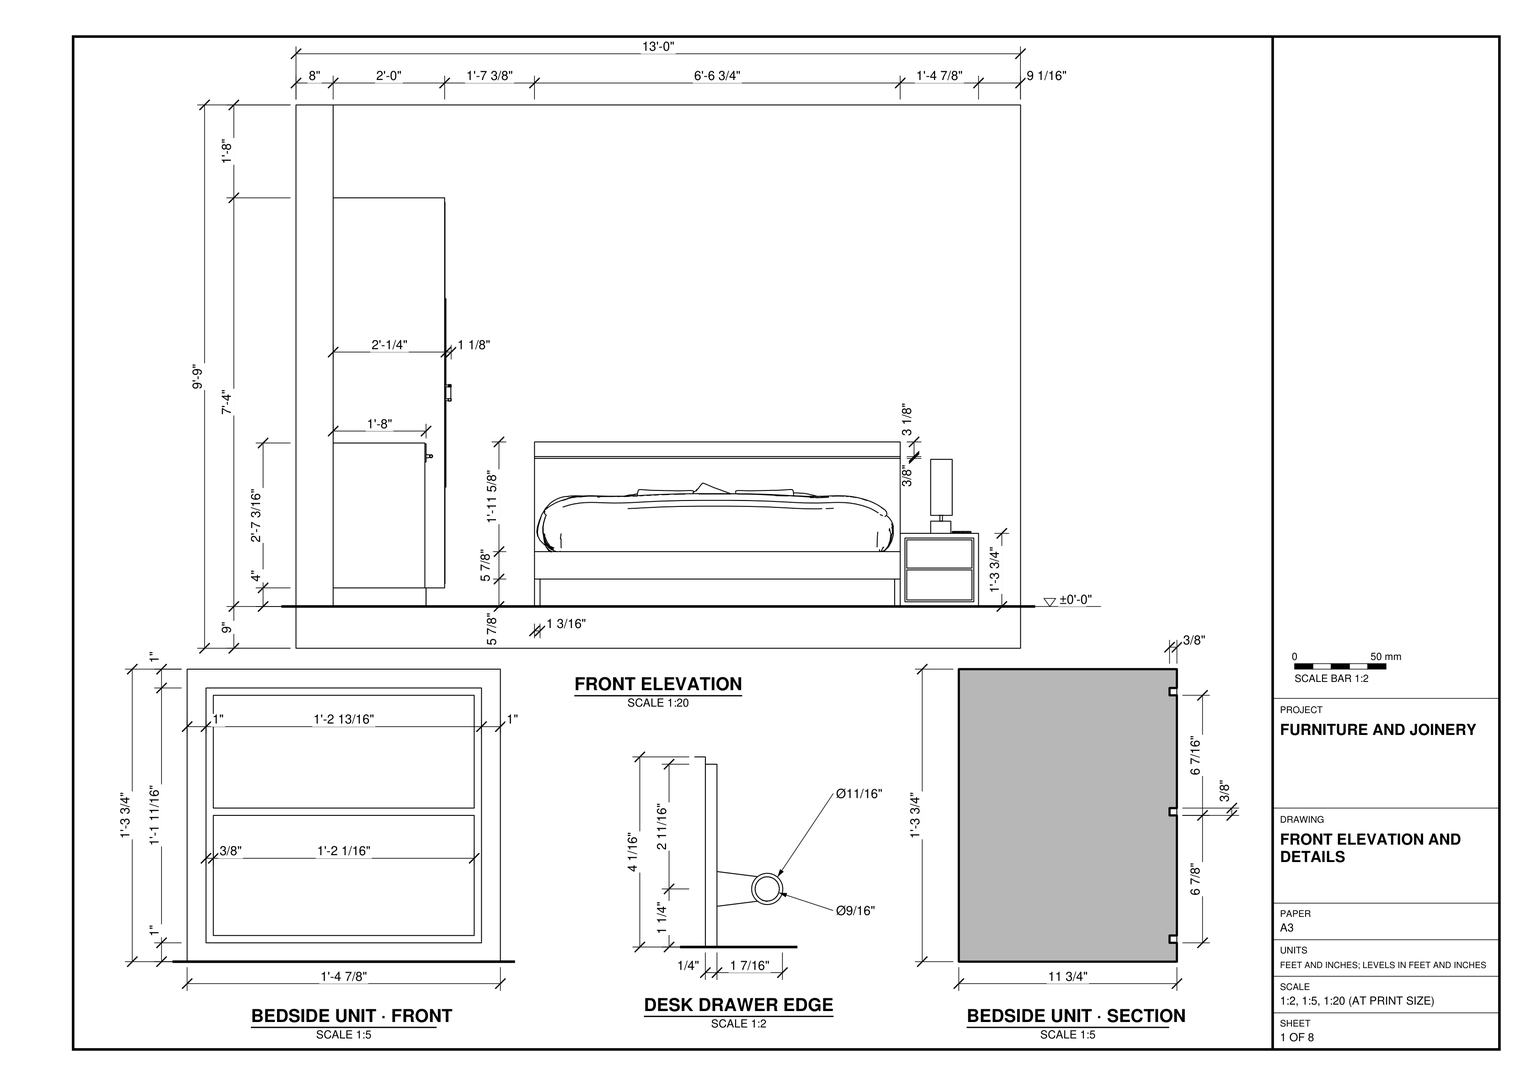
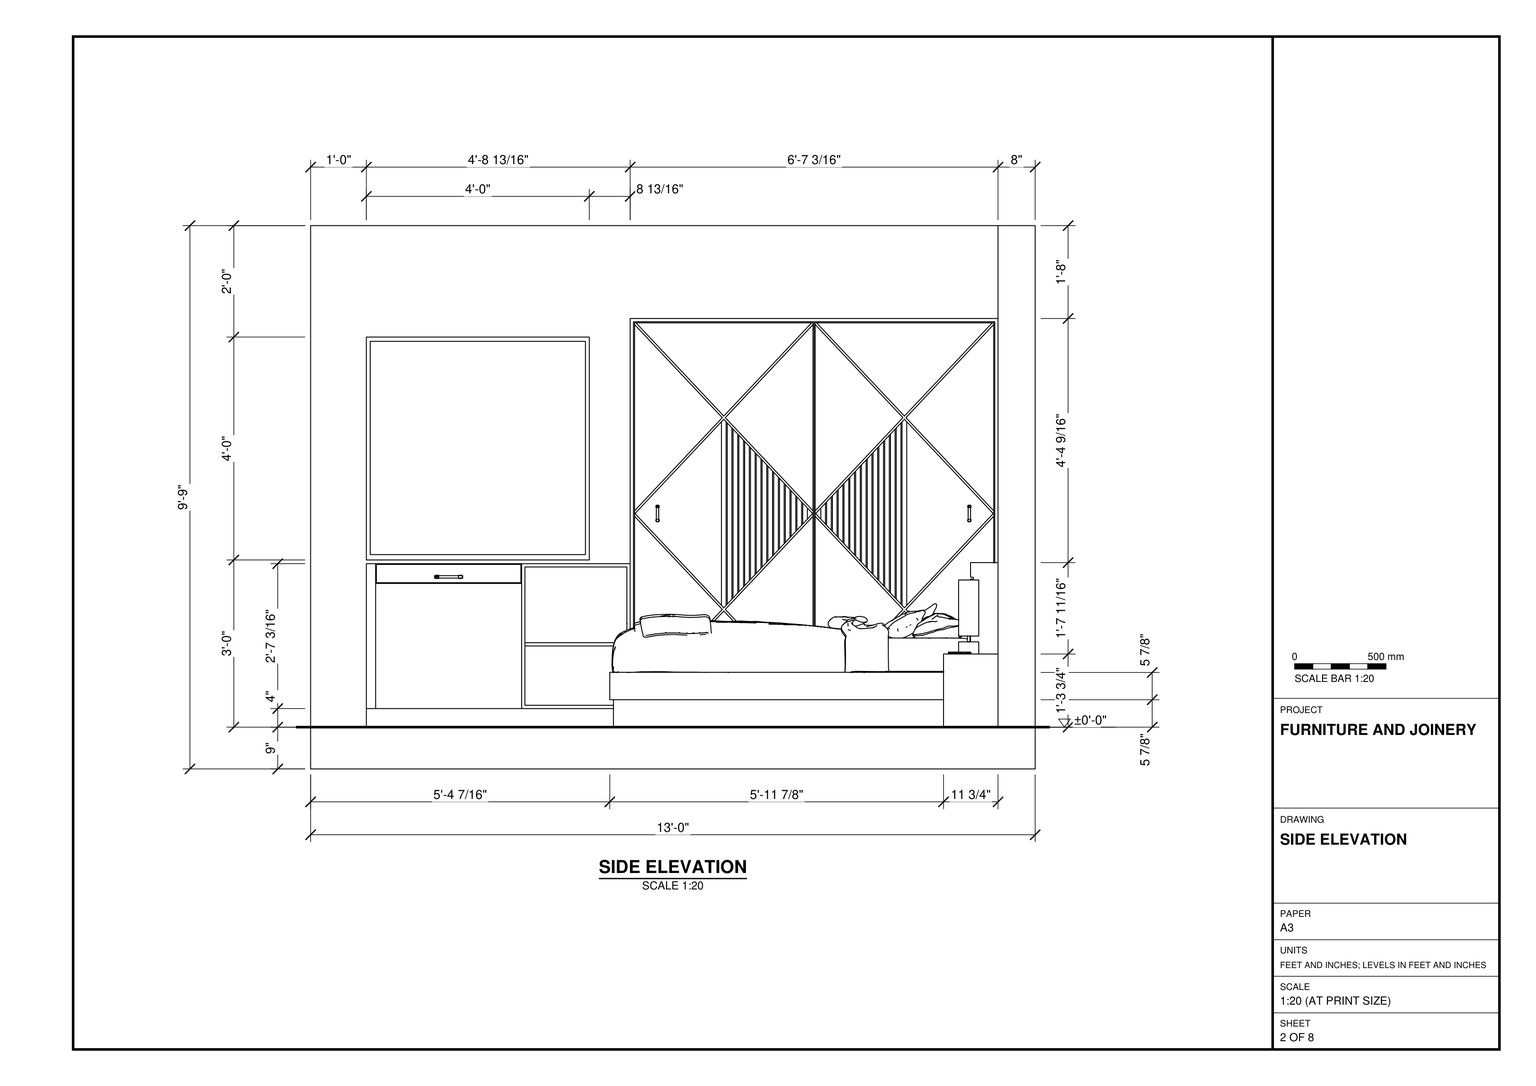
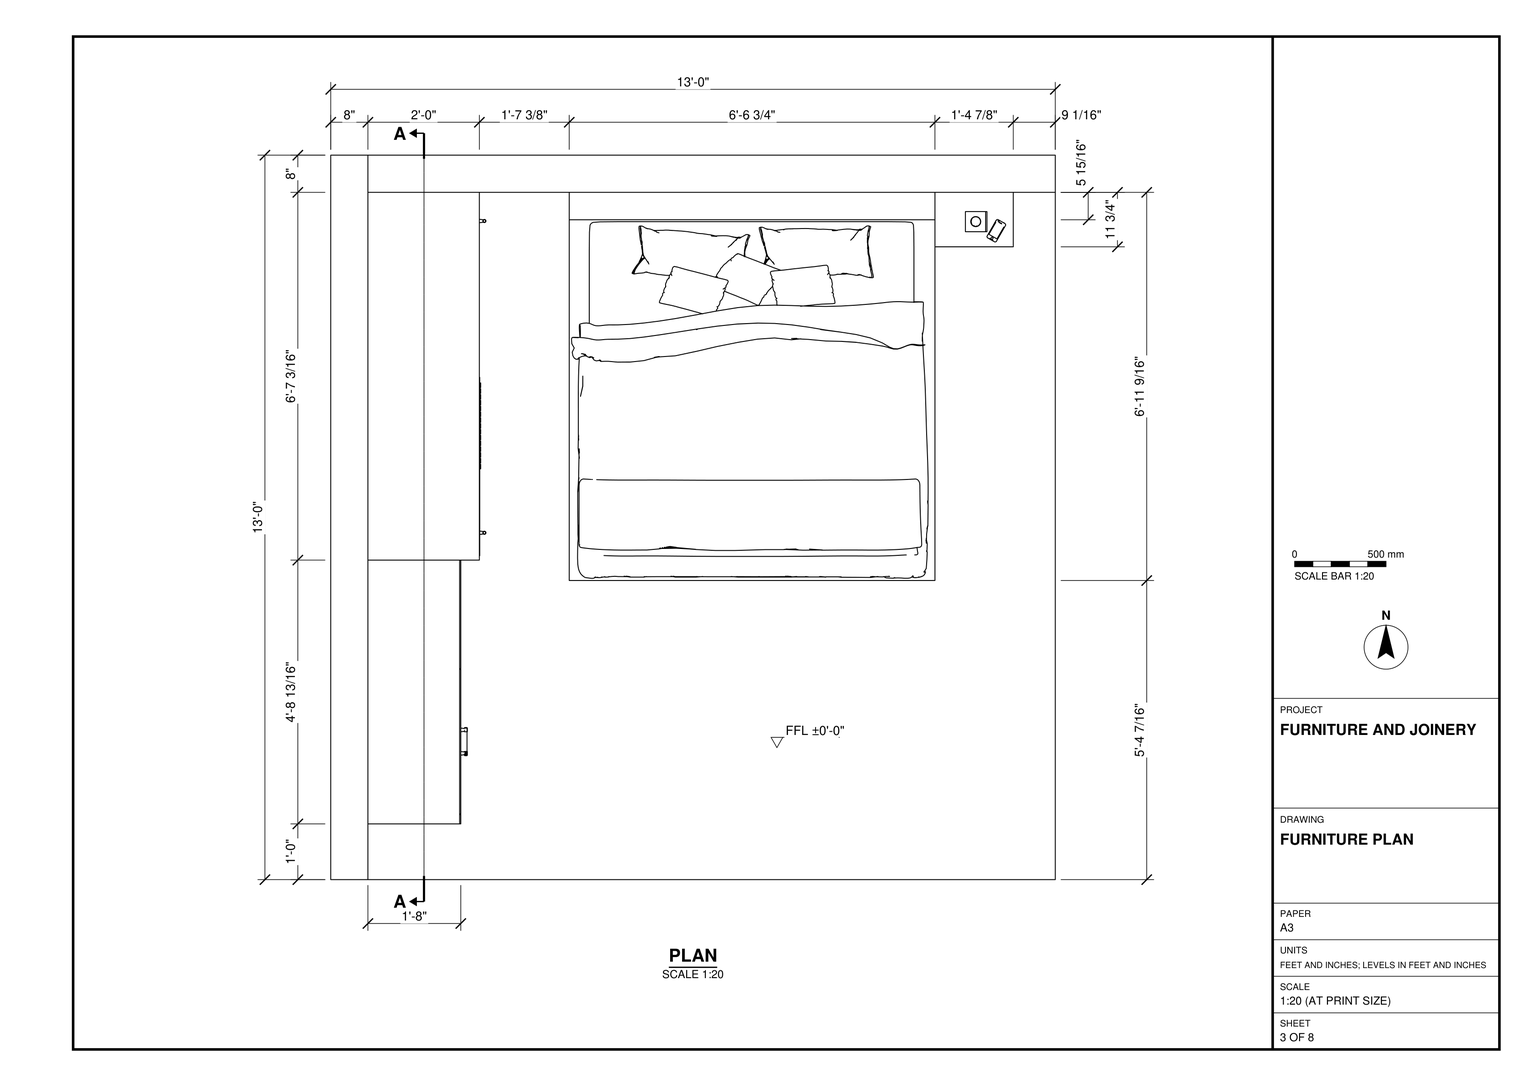
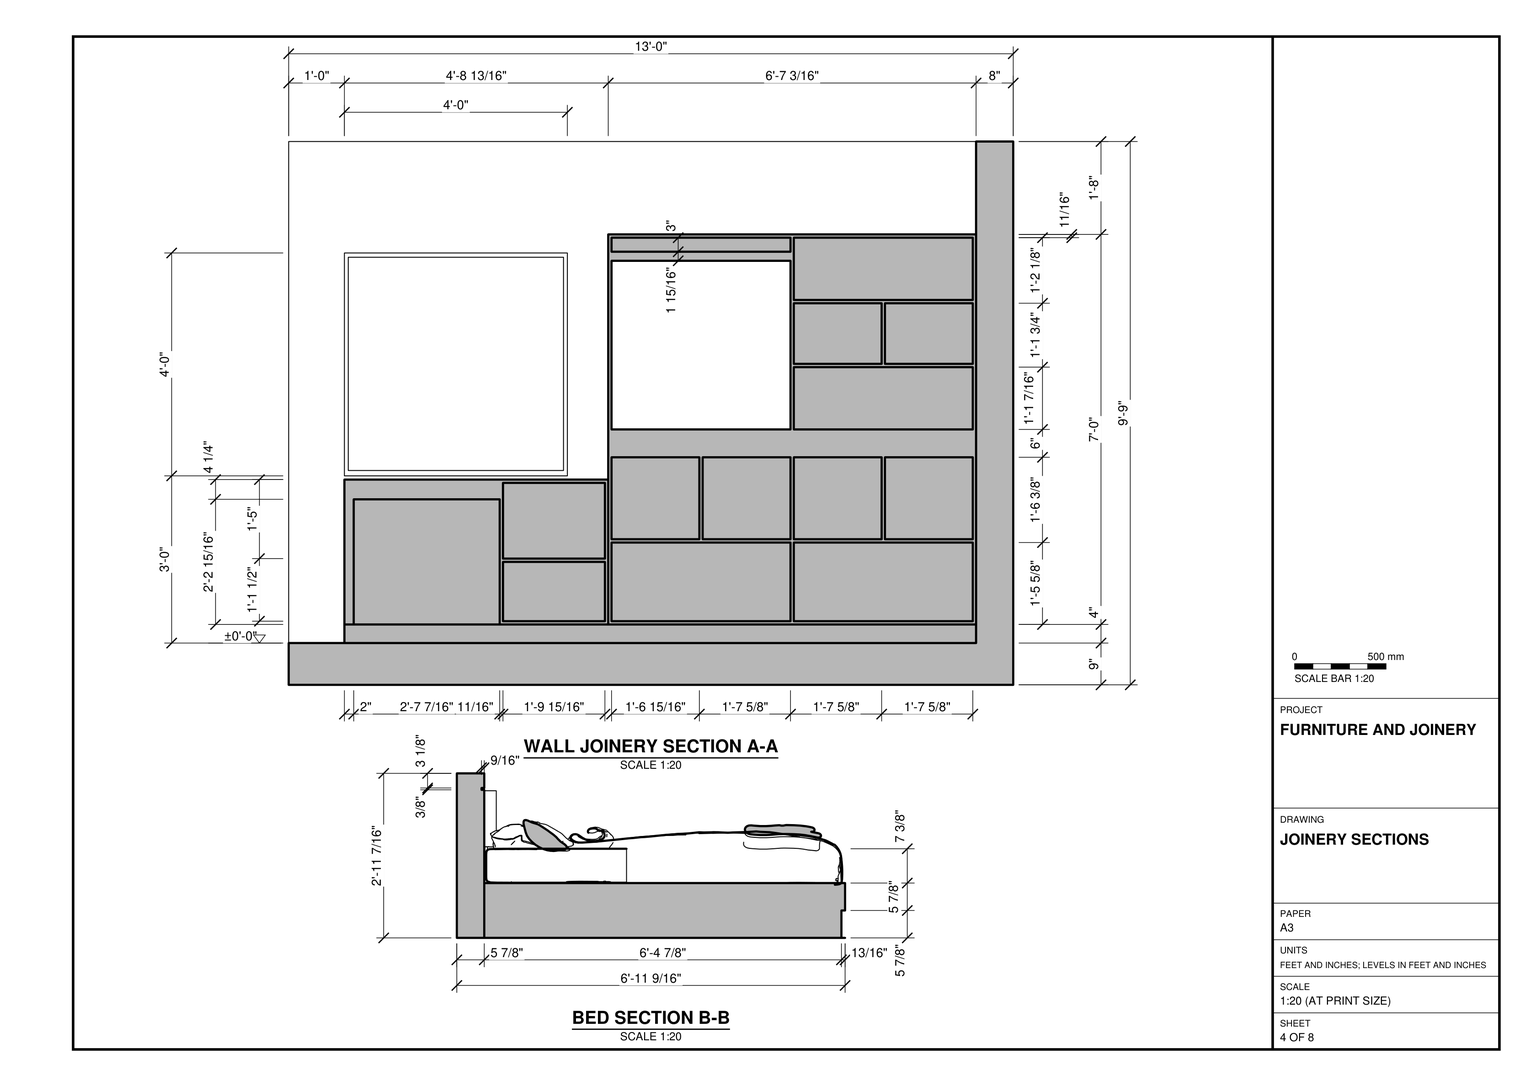
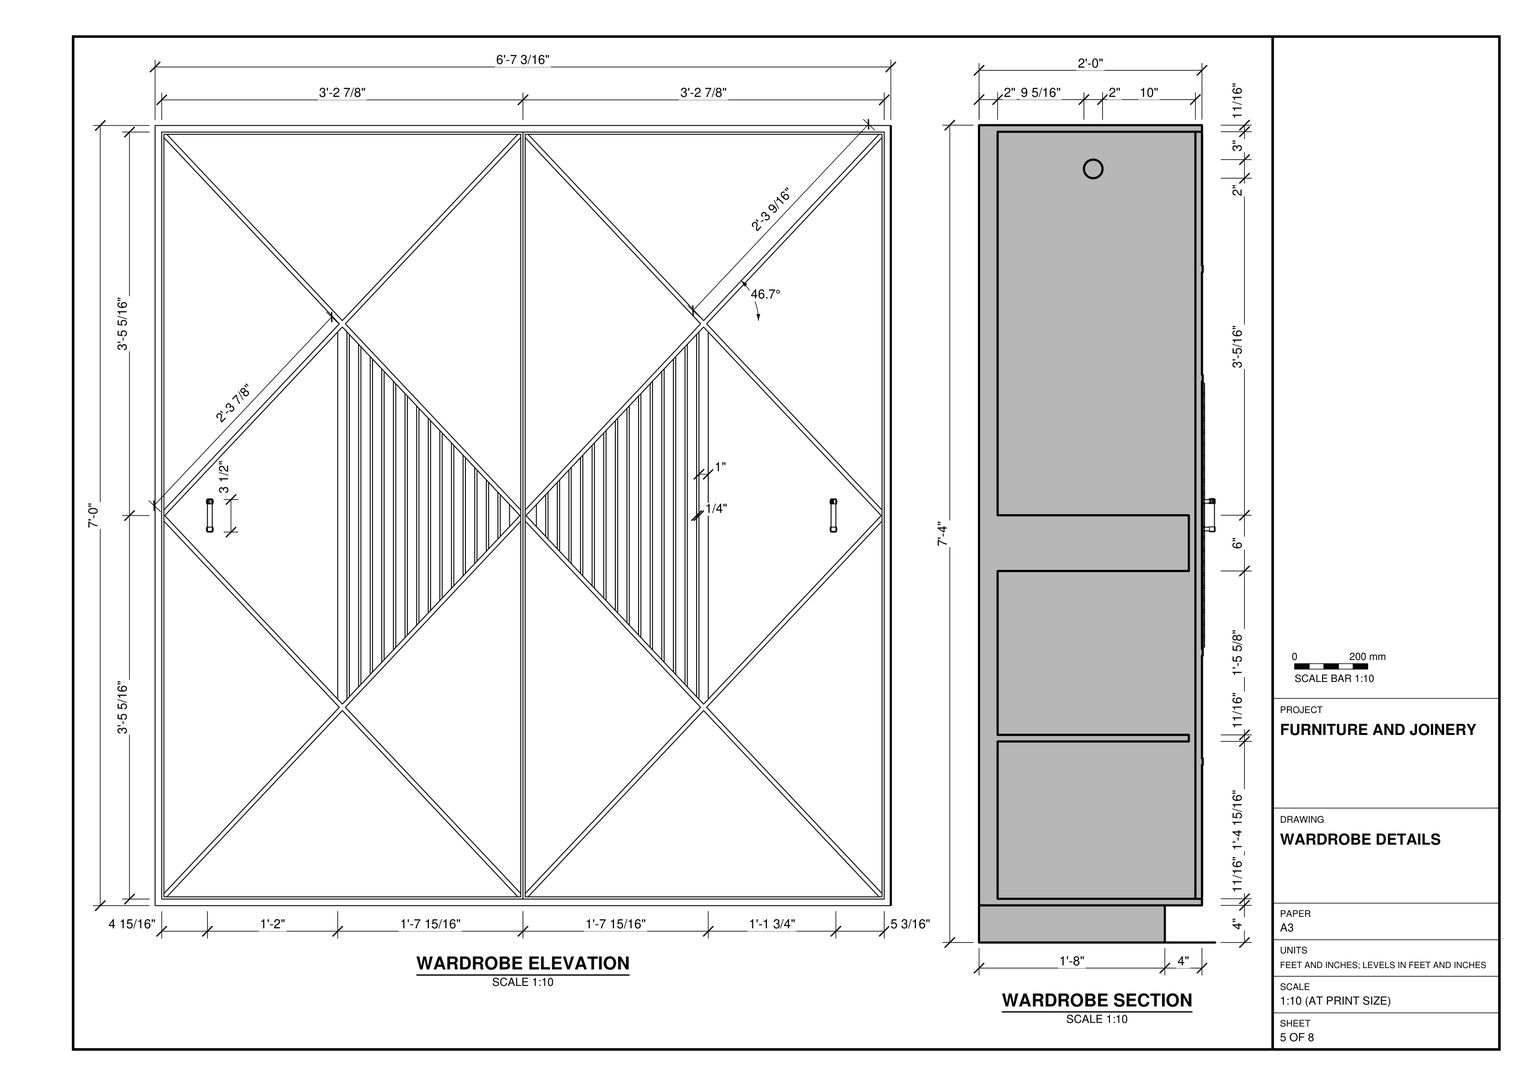
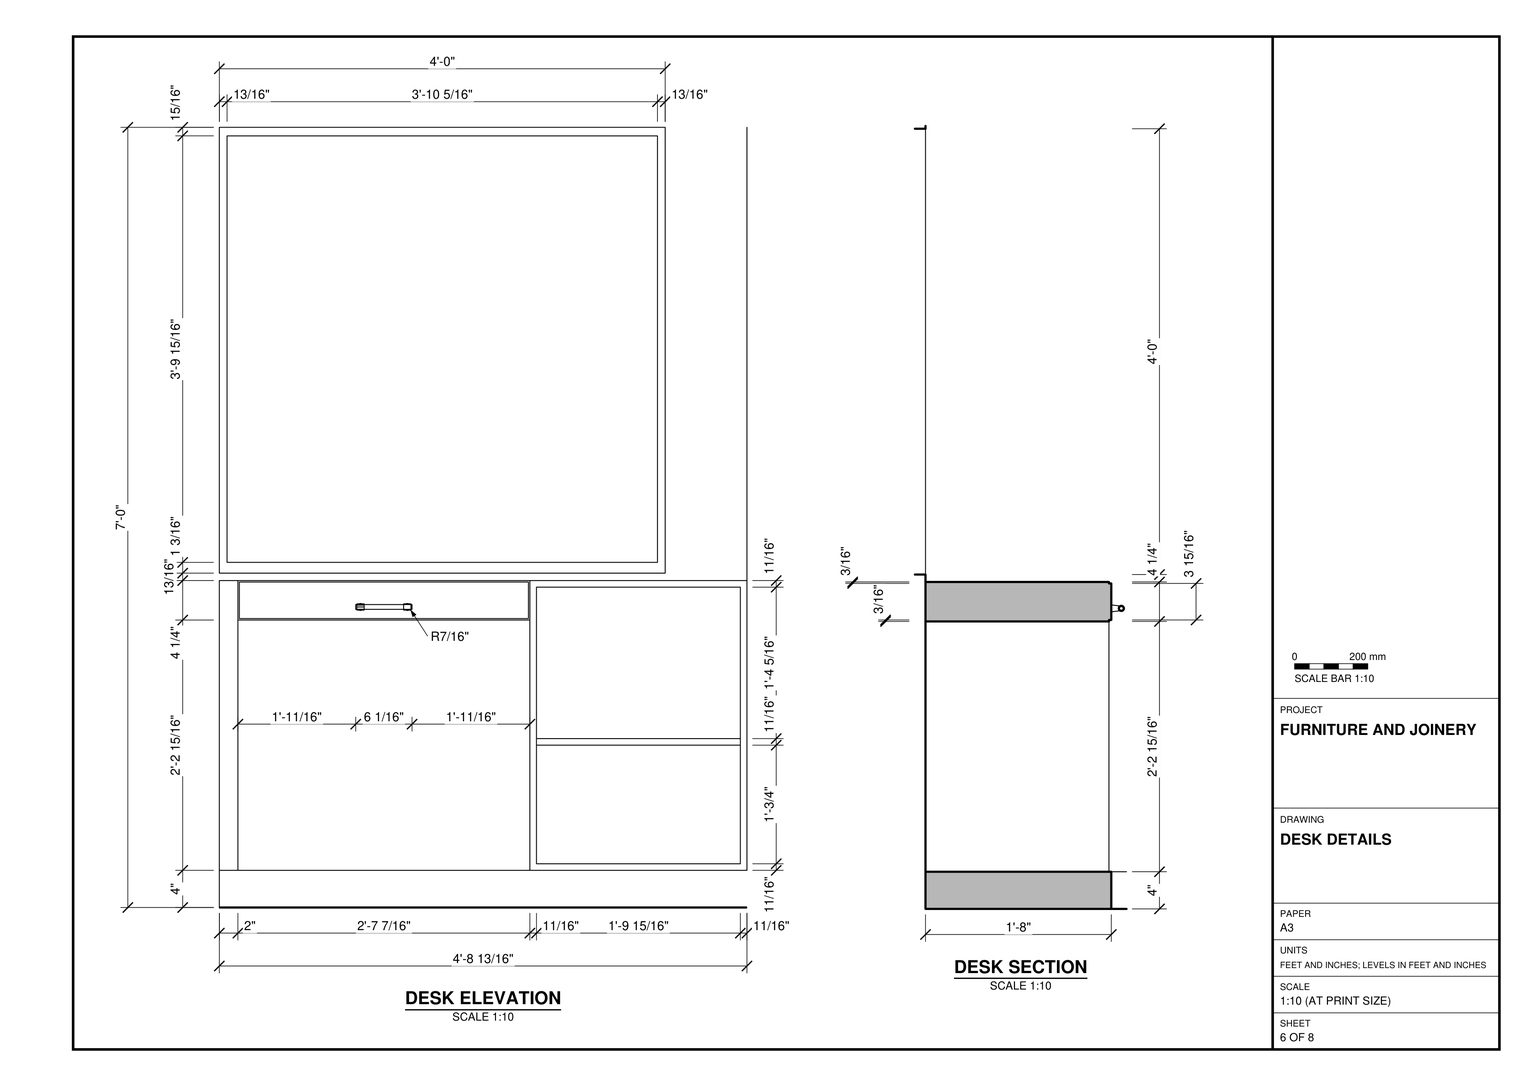
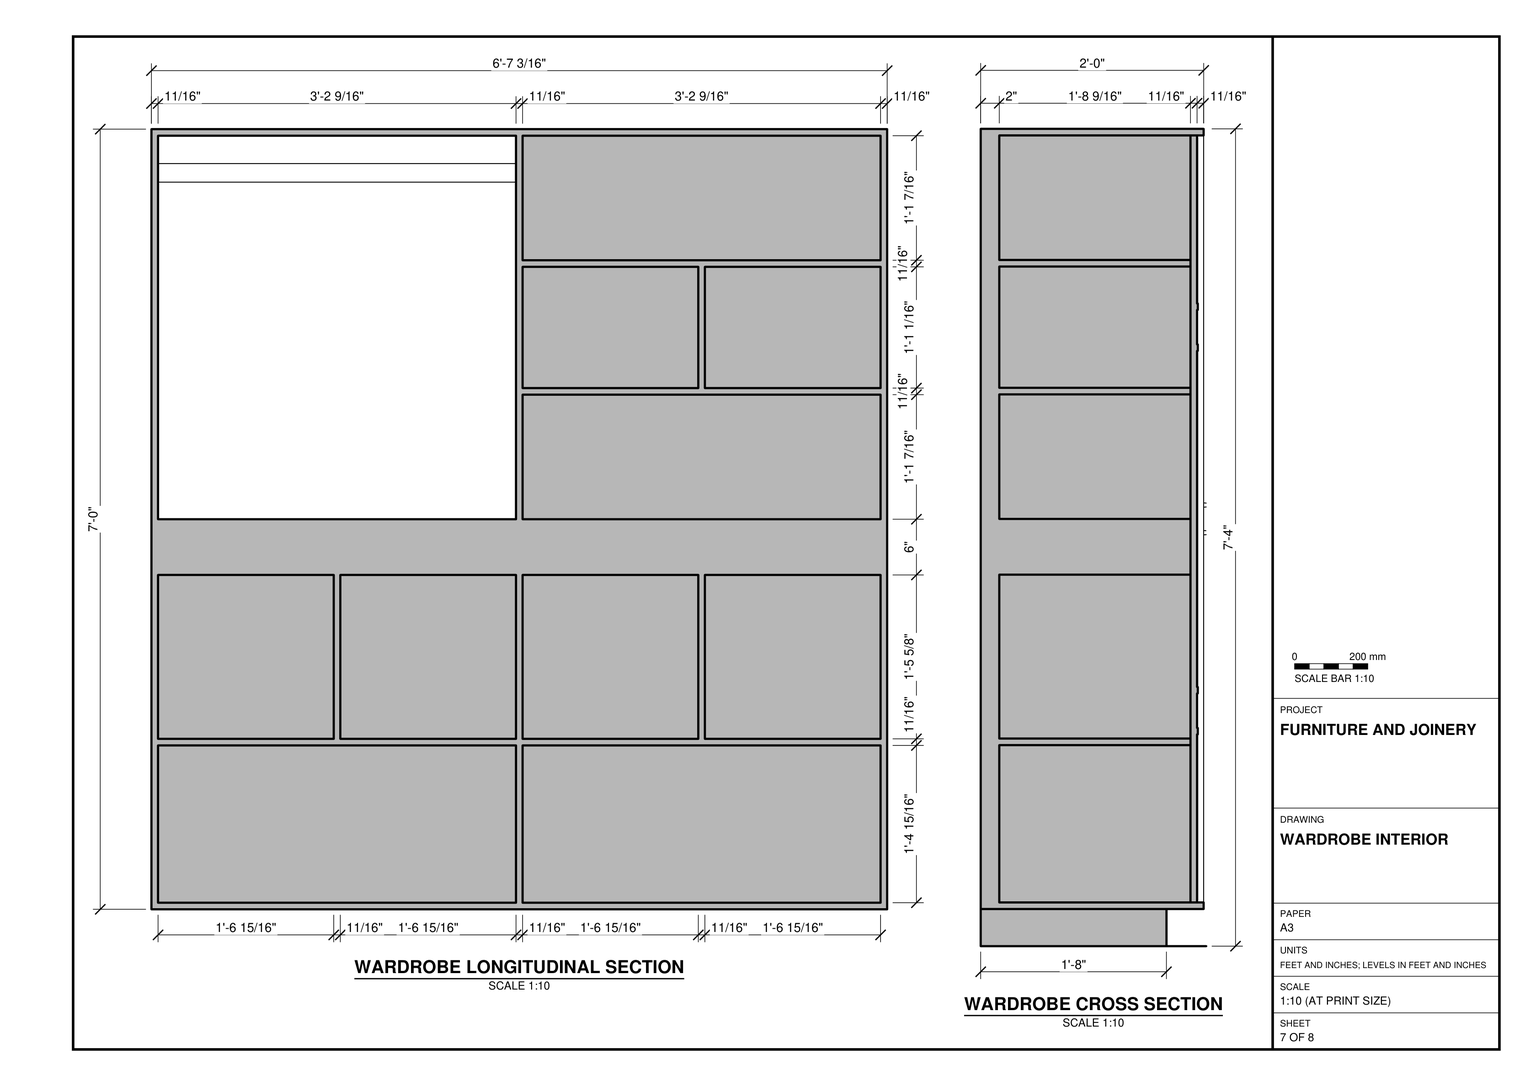
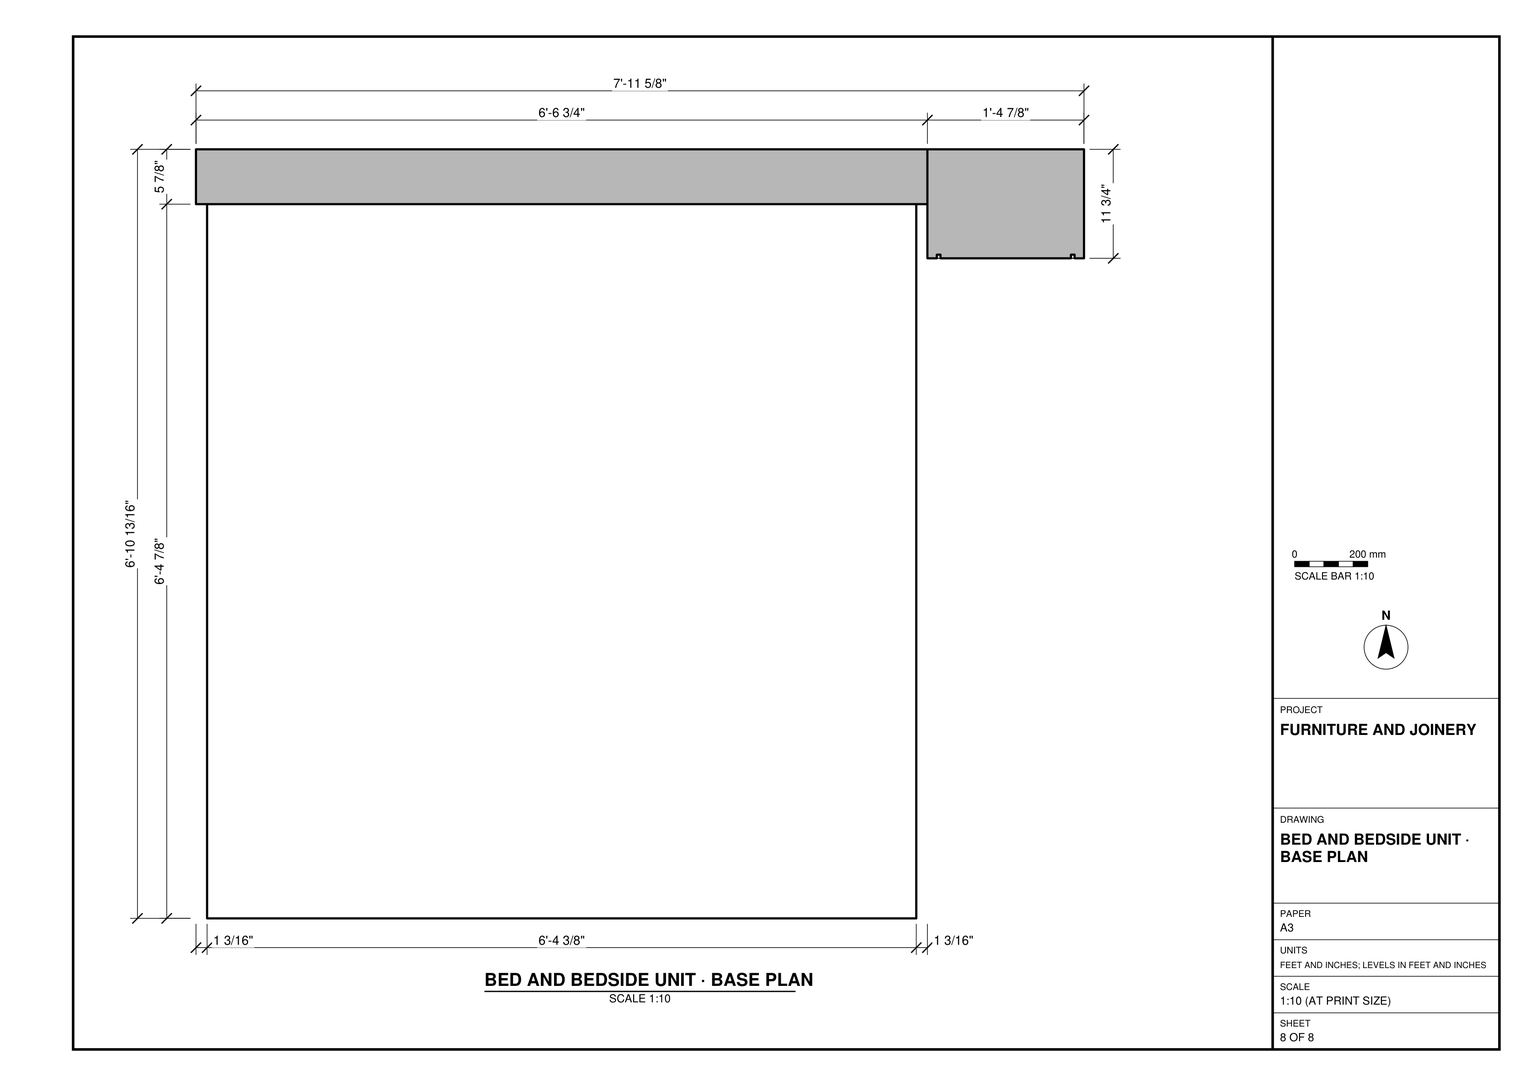
Build the bedroom interior in SketchUp from task_files/diagram_01.pdf. Work in feet and inches. The overall footprint is 13'-0" by 13'-0", and the overall height is 9'-9", measured from the underside of the slab. Set the finished floor at ±0'-0". Model the 9" floor slab and the 8" walls along the north and west edges shown in plan, leaving the other two sides open.

Place the headboard against the north wall, with the platform bed extending south and the bedside unit immediately to the right of the headboard. Use the elevations to shape the bed base and the detail views to set out the two recessed fronts of the bedside unit. Run the wardrobe along the west wall from the northwest corner. Reproduce the diagonal divisions, striped triangular fields and pulls on its paired fronts. Continue south along the same wall with the shallower desk, including its drawer, knee space, storage bay and square framed panel above.

Keep the walls, slab and each furniture or joinery piece in separate groups or components, and use components for repeated parts. Decor and loose items, including the bedside lamp and cushions, may be any suitable library components. Save the completed SketchUp model as output_files/bedroom_with_a_platform_bed_and_fitted_joinery.skp.

# SketchUp Ruby script. Lengths in inches.
U = 1.inch
M = Sketchup.active_model
def pt(a) = Geom::Point3d.new(a.map { |v| v * U })
def face(e, loops, mat)
  f = e.add_face(loops[0].map { |a| pt(a) })
  loops[1..].each { |l| e.add_face(l.map { |a| pt(a) }).erase! }
  f.material = f.back_material = mat if mat
  f
end
# faces: each face lists its corners as indices into pts; further lists are holes
def faces(e, pts, list, mat = nil) = list.each { |f| face(e, (f[0].is_a?(Array) ? f : [f]).map { |l| l.map { |i| pts[i] } }, mat) }
# xy, xz, yz: faces in a plane at the given z, y or x. An outline is a flat list of corners, or four numbers for a rectangle; further outlines are holes
def ring(l) = l.size == 4 ? [[l[0], l[1]], [l[2], l[1]], [l[2], l[3]], [l[0], l[3]]] : l.each_slice(2).to_a
def flat(e, list, mat, &to3) = list.each { |f| face(e, (f[0].is_a?(Array) ? f : [f]).map { |l| ring(l).map { |u, v| to3.(u, v) } }, mat) }
def xy(e, z, list, mat = nil) = flat(e, list, mat) { |x, y| [x, y, z] }
def xz(e, y, list, mat = nil) = flat(e, list, mat) { |x, z| [x, y, z] }
def yz(e, x, list, mat = nil) = flat(e, list, mat) { |y, z| [x, y, z] }
def lines(e, pts, list) = list.each { |a, b| e.add_line(pt(pts[a]), pt(pts[b])) }
# prism: a flat outline (further loops are holes) pulled along v
def prism(e, loops, v, mat = nil)
  f = face(e, loops, mat); d = Geom::Vector3d.new(v.map { |x| x * U })
  f.pushpull(f.normal.samedirection?(d) ? d.length : -d.length)
end
def box(e, o, s, mat = nil) = prism(e, [[o, [o[0] + s[0], o[1], o[2]], [o[0] + s[0], o[1] + s[1], o[2]], [o[0], o[1] + s[1], o[2]]]], [0, 0, s[2]], mat)
def at(x, y, z, deg = 0) = Geom::Transformation.translation(pt([x, y, z])) * Geom::Transformation.rotation(ORIGIN, Z_AXIS, deg.degrees)
def axes(o, x, y, z) = Geom::Transformation.new([*x, 0, *y, 0, *z, 0, *pt(o).to_a, 1])
def part(name) = M.definitions.add(name)
# library, detail: a bought-in or finely detailed component or shape, given as its bounding box
def library(name, o, s) = part(name).tap { |d| box(d.entities, o, s) }
def detail(e, o, s) = box(e.add_group.entities, o, s)
def put(e, d, t, mat = nil) = e.add_instance(d, t).tap { |i| i.material = mat if mat }
def group(e, t, mat = nil) = e.add_group.tap { |g| g.transformation = t; g.material = mat if mat }.entities
root = M.entities
M.materials.add("[0043_SaddleBrown]").color = [139, 69, 19]
M.materials.add("[0044_DarkGoldenrod]").color = [184, 134, 11]
M.materials.add("[0119_RosyBrown]").color = [188, 143, 143]
M.materials.add("[0136_Charcoal]").color = [35, 35, 35]
M.materials.add("[Color E01]").color = [255, 255, 204]
M.materials.add("[Color M00]").color = [255, 255, 255]
M.materials.add("[Slate Light Tile]").color = [54, 54, 54]
M.materials.add("[Tile Checker BW]").color = [125, 112, 107]
M.materials.add("[Translucent_Glass_Blue]").color = [100, 149, 237]
M.materials["[Translucent_Glass_Blue]"].alpha = 0.5
M.materials.add("[Wood Veneer 01]").color = [120, 70, 37]
M.materials.add("[Wood_Bamboo_Medium]").color = [177, 105, 43]
c1 = library("Platform bed",[0,0,0],[83.59,95.6,35.43])
c2 = part("Untitled")
xy(c2.entities,34.68,[[46.57,0,194.75,6.75]])
xy(c2.entities,36.94,[[49.13,0,192.19,6.75]],"[Wood_Bamboo_Medium]")
xy(c2.entities,126.69,[[49.13,0,192.19,6.75]],"[Wood_Bamboo_Medium]")
xy(c2.entities,128.49,[[46.57,0,194.75,6.75]],"[Wood_Bamboo_Medium]")
xz(c2.entities,0,[[49.13,36.94,192.19,126.69]],"[Translucent_Glass_Blue]")
xz(c2.entities,0,[[[46.57,34.68,194.75,128.49],[49.13,36.94,192.19,126.69]]],"[Wood_Bamboo_Medium]")
xz(c2.entities,6.75,[[49.13,36.94,192.19,126.69]],"[Translucent_Glass_Blue]")
xz(c2.entities,6.75,[[[46.57,34.68,194.75,128.49],[49.13,36.94,192.19,126.69]]],"[Wood_Bamboo_Medium]")
yz(c2.entities,46.57,[[0,34.68,6.75,128.49]],"[Wood_Bamboo_Medium]")
yz(c2.entities,49.13,[[0,36.94,6.75,126.69]],"[Wood_Bamboo_Medium]")
yz(c2.entities,192.19,[[0,36.94,6.75,126.69]],"[Wood_Bamboo_Medium]")
yz(c2.entities,194.75,[[0,34.68,6.75,128.49]])
c3 = library("1-POIGNEE CLC2\#1",[-3.03,-0.375,0],[6.06,0.75,1.42])
c4 = library("Group\#2",[128,-0.28,0],[77.78,1.7,82.58])
put(root,c1,at(146.95,64.41,9,90))
put(root,c2,axes([5.625,-3.08,27.26],[0,0.32391,0],[-0.62,0,0],[0,0,0.51166]))
g1 = group(root,at(0,0,0))
xy(g1,0,[[0,0,156,156]])
xy(g1,9,[[8,0,156,148]],"[Tile Checker BW]")
xy(g1,45,[[0,12,8,60]])
xy(g1,93,[[0,12,8,60]])
xy(g1,117,[[0,0,8,156],[8,148,156,156]])
xz(g1,0,[[0,0,156,0,156,9,8,9,8,117,0,117]])
xz(g1,12,[[0,45,8,93]])
xz(g1,60,[[0,45,8,93]])
xz(g1,148,[[8,9,156,117]],"[0119_RosyBrown]")
xz(g1,156,[[0,0,156,117]])
yz(g1,0,[[[0,0,156,117],[12,45,60,93]]])
yz(g1,8,[[[0,9,148,117],[12,45,60,93]]],"[0119_RosyBrown]")
yz(g1,156,[[0,0,156,0,156,117,148,117,148,9,0,9]])
g2 = group(root,at(8,68.01,9))
detail(g2,[24,6.31,44.22],[1.42,0.75,3.58])
detail(g2,[24,73.44,44.22],[1.42,0.75,3.58])
g3 = group(g2,at(24,0.79,0,90))
xy(g3,0,[[-56.8,4,79.2,24]])
xy(g3,4,[[0,4,79.2,24]])
xy(g3,4,[[-56.8,4,-54.8,4.25],[-23.37,4,0,4.25]],"[Color M00]")
xy(g3,4,[[-54.8,4,-23.37,24],[-56.8,4.25,-54.8,24],[-23.37,4.25,0,24]],"[Slate Light Tile]")
xy(g3,4,[[0,0,79.2,4]],"[Wood Veneer 01]")
xy(g3,4.71,[[0.71,0,78.49,0.71],[0.71,0.71,78.49,1.42],[0.71,1.42,39.25,22],[39.95,1.42,78.49,22]])
xy(g3,4.71,[[-22.66,4.25,-0.71,24]],"[0136_Charcoal]")
xy(g3,17.47,[[-22.66,4.25,-0.71,24]],"[0136_Charcoal]")
xy(g3,18.18,[[-22.66,4.25,-0.71,24]],"[0136_Charcoal]")
xy(g3,21.65,[[0.71,1.42,19.62,22],[19.62,1.42,20.33,22],[20.33,1.42,39.25,22],[39.95,1.42,58.87,22],[58.87,1.42,59.58,22],
  [59.58,1.42,78.49,22]])
xy(g3,22.35,[[0.71,1.42,19.62,22],[20.33,1.42,39.25,22],[39.95,1.42,58.87,22],[59.58,1.42,78.49,22]])
xy(g3,30.95,[[-54.8,4.25,-23.37,24]],"[Color M00]")
xy(g3,31.11,[[-54.64,4,-23.52,4.25]],"[Color M00]")
xy(g3,34.49,[[-22.66,4.25,-0.71,24]],"[0136_Charcoal]")
xy(g3,35.04,[[-54.64,4,-23.52,4.25]],"[Color M00]")
xy(g3,35.2,[[-56.8,4.25,0,24]],"[0043_SaddleBrown]")
xy(g3,40,[[0.71,1.42,19.62,22],[20.33,1.42,39.25,22],[39.95,1.42,58.87,22],[59.58,1.42,78.49,22]])
xy(g3,46,[[0.71,1.42,39.25,22],[39.95,1.42,78.49,22]])
xy(g3,59.41,[[39.95,1.42,58.87,22],[58.87,1.42,59.58,22],[59.58,1.42,78.49,22]])
xy(g3,60.12,[[39.95,1.42,58.87,22],[59.58,1.42,78.49,22]])
xy(g3,73.17,[[39.95,1.42,58.87,22],[59.58,1.42,78.49,22]])
xy(g3,73.88,[[39.95,1.42,59.22,22],[59.22,1.42,78.49,22]])
xy(g3,82.29,[[0.71,11.65,39.25,11.71],[0.71,11.71,39.25,11.77]])
xy(g3,84.29,[[0.71,11.65,39.25,11.71],[0.71,11.71,39.25,11.77]])
xy(g3,87.29,[[0.71,0,78.49,0.71],[0.71,0.71,78.49,1.42],[0.71,1.42,39.25,22],[39.95,1.42,78.49,22]])
xy(g3,88,[[0,0,79.2,24]],"[Wood Veneer 01]")
xz(g3,0,[[[0,4,79.2,88],[0.71,4.71,78.49,87.29]]],"[Wood Veneer 01]")
xz(g3,1.42,[[39.25,4.71,39.95,87.29],[0.71,21.65,39.25,21.65,39.25,22.35,20.33,22.35,20.33,40,19.62,40,19.62,22.35,0.71,22.35],[39.95,21.65,78.49,21.65,78.49,22.35,59.58,22.35,59.58,40,58.87,40,58.87,22.35,39.95,22.35],[[0.71,40,39.25,46],[0.83,40.12,19.86,45.88],[20.1,40.12,39.13,45.88]],[[39.95,40,78.49,46],[59.34,40.12,78.375,45.88],[40.07,40.12,59.1,45.88]],
  [0.83,40.12,19.86,45.88],[20.1,40.12,39.13,45.88],[40.07,40.12,59.1,45.88],[59.34,40.12,78.375,45.88],[39.95,59.41,78.49,60.12],
  [58.87,60.12,59.58,73.17],[39.95,73.17,78.49,73.88]])
xz(g3,4,[[-54.64,31.11,-23.52,35.04]],"[0044_DarkGoldenrod]")
xz(g3,4,[[-56.8,0,79.2,4]],"[Slate Light Tile]")
xz(g3,4.25,[[-56.8,4,-54.8,35.2],[[-23.37,4,0,35.2],[-22.66,4.71,-0.71,34.49]],[-22.66,17.47,-0.71,18.18]],"[0043_SaddleBrown]")
xz(g3,4.25,[[[-54.8,30.95,-23.37,35.2],[-54.64,31.11,-23.52,35.04]]],"[Color M00]")
xz(g3,10.71,[[0.71,83.23,39.25,83.29],[0.71,83.29,39.25,83.35]])
xz(g3,12.71,[[0.71,83.23,39.25,83.29],[0.71,83.29,39.25,83.35]])
xz(g3,22,[[0.71,4.71,39.25,21.65],[39.95,4.71,78.49,21.65],[0.71,22.35,19.62,40],[20.33,22.35,39.25,40],[39.95,22.35,58.87,40],
  [59.58,22.35,78.49,40],[0.71,46,39.25,87.29],[39.95,46,78.49,59.41],[39.95,60.12,58.87,73.17],[59.58,60.12,78.49,73.17],
  [39.95,73.88,78.49,87.29]])
xz(g3,24,[[-56.8,0,79.2,4],[0,4,79.2,88]])
xz(g3,24,[[[-56.8,4,-56.8,35.2,0,35.2,0,4,-23.37,4,-23.37,30.95,-54.8,30.95,-54.8,4],[-22.66,18.18,-0.71,34.49],[-22.66,4.71,-0.71,17.47]]],"[Slate Light Tile]")
yz(g3,-56.8,[[4.25,4,24,35.2]],"[0043_SaddleBrown]")
yz(g3,-56.8,[[4,0,24,4]],"[Slate Light Tile]")
yz(g3,-54.8,[[4.25,4,24,30.95]],"[0043_SaddleBrown]")
yz(g3,-54.64,[[4,31.11,4.25,35.04]],"[Color M00]")
yz(g3,-23.52,[[4,31.11,4.25,35.04]],"[Color M00]")
yz(g3,-23.37,[[4.25,4,24,30.95]],"[0043_SaddleBrown]")
yz(g3,-22.66,[[4.25,4.71,24,17.47],[4.25,18.18,24,30.95],[4.25,30.95,24,34.49]],"[0136_Charcoal]")
yz(g3,-0.71,[[4.25,4.71,24,17.47],[4.25,18.18,24,34.49]],"[0136_Charcoal]")
yz(g3,0,[[4.25,4,24,35.2]],"[Slate Light Tile]")
yz(g3,0,[[0,4,0,88,24,88,24,35.2,4.25,35.2,4.25,4]],"[Wood Veneer 01]")
yz(g3,0.71,[[0,4.71,0.71,87.29],[0.71,4.71,1.42,87.29],[1.42,4.71,22,21.65],[1.42,22.35,22,40],[[1.42,46,22,87.29],[11.65,82.29,11.58,82.3,11.46,82.32,11.34,82.36,11.28,82.39,11.23,82.42,11.17,82.45,11.12,82.48,11.07,82.52,11.02,82.5625,10.98,82.61,10.9375,82.65,10.9,82.7,10.86,82.76,10.83,82.81,10.8,82.87,10.78,82.92,10.74,83.04,10.73,83.1,10.72,83.17,10.71,83.23,10.71,83.35,10.72,83.42,10.74,83.54,10.8,83.72,10.83,83.77,10.86,83.83,10.9,83.88,10.9375,83.93,10.98,83.98,11.02,84.02,11.07,84.0625,11.12,84.1,11.17,84.14,11.23,84.17,11.28,84.2,11.46,84.26,11.58,84.28,11.65,84.29,11.77,84.29,11.83,84.28,11.9,84.27,11.96,84.26,12.08,84.22,12.13,84.2,12.19,84.17,12.24,84.14,12.3,84.1,12.35,84.0625,12.39,84.02,12.4375,83.98,12.48,83.93,12.52,83.88,12.55,83.83,12.58,83.77,12.61,83.72,12.64,83.66,12.68,83.54,12.7,83.42,12.71,83.35,12.71,83.23,12.7,83.17,12.69,83.1,12.68,83.04,12.64,82.92,12.61,82.87,12.58,82.81,12.55,82.76,12.52,82.7,12.48,82.65,12.4375,82.61,12.39,82.5625,12.35,82.52,12.3,82.48,12.24,82.45,12.19,82.42,12.13,82.39,12.08,82.36,11.96,82.32,11.9,82.31,11.83,82.3,11.77,82.29]]])
yz(g3,19.62,[[1.42,22.35,22,40]])
yz(g3,20.33,[[1.42,22.35,22,40]])
yz(g3,39.25,[[1.42,4.71,22,21.65],[1.42,22.35,22,40],[[1.42,46,22,87.29],[11.65,82.29,11.77,82.29,11.83,82.3,11.9,82.31,11.96,82.32,12.08,82.36,12.13,82.39,12.19,82.42,12.24,82.45,12.3,82.48,12.35,82.52,12.39,82.5625,12.4375,82.61,12.48,82.65,12.52,82.7,12.55,82.76,12.58,82.81,12.61,82.87,12.64,82.92,12.68,83.04,12.69,83.1,12.7,83.17,12.71,83.23,12.71,83.35,12.7,83.42,12.68,83.54,12.64,83.66,12.61,83.72,12.58,83.77,12.55,83.83,12.52,83.88,12.48,83.93,12.4375,83.98,12.39,84.02,12.35,84.0625,12.3,84.1,12.24,84.14,12.19,84.17,12.13,84.2,12.08,84.22,11.96,84.26,11.9,84.27,11.83,84.28,11.77,84.29,11.65,84.29,11.58,84.28,11.46,84.26,11.28,84.2,11.23,84.17,11.17,84.14,11.12,84.1,11.07,84.0625,11.02,84.02,10.98,83.98,10.9375,83.93,10.9,83.88,10.86,83.83,10.83,83.77,10.8,83.72,10.74,83.54,10.72,83.42,10.71,83.35,10.71,83.23,10.72,83.17,10.73,83.1,10.74,83.04,10.78,82.92,10.8,82.87,10.83,82.81,10.86,82.76,10.9,82.7,10.9375,82.65,10.98,82.61,11.02,82.5625,11.07,82.52,11.12,82.48,11.17,82.45,11.23,82.42,11.28,82.39,11.34,82.36,11.46,82.32,11.58,82.3]]])
yz(g3,39.95,[[1.42,4.71,22,21.65],[1.42,22.35,22,40],[1.42,46,22,59.41],[1.42,60.12,22,73.17],[1.42,73.88,22,87.29]])
yz(g3,58.87,[[1.42,22.35,22,40],[1.42,60.12,22,73.17]])
yz(g3,59.58,[[1.42,22.35,22,40],[1.42,60.12,22,73.17]])
yz(g3,78.49,[[0,4.71,0.71,87.29],[0.71,4.71,1.42,87.29],[1.42,4.71,22,21.65],[1.42,22.35,22,40],[1.42,46,22,59.41],
  [1.42,60.12,22,73.17],[1.42,73.88,22,87.29]])
yz(g3,79.2,[[4,0,24,4]],"[Slate Light Tile]")
yz(g3,79.2,[[0,4,24,88]],"[Wood Veneer 01]")
p = [[0.71,11.34,82.36],[0.71,11.4,82.34],[39.25,11.4,82.34],[39.25,11.34,82.36],[0.71,11.46,82.32],[39.25,11.46,82.32],
  [0.71,11.52,82.31],[39.25,11.52,82.31],[0.71,11.58,82.3],[39.25,11.58,82.3],[0.71,11.65,82.29],[39.25,11.65,82.29],
  [0.71,11.77,82.29],[0.71,11.83,82.3],[39.25,11.83,82.3],[39.25,11.77,82.29],[0.71,11.9,82.31],[39.25,11.9,82.31],
  [0.71,11.96,82.32],[39.25,11.96,82.32],[0.71,12.02,82.34],[39.25,12.02,82.34],[0.71,12.08,82.36],[39.25,12.08,82.36],
  [0.71,11.12,82.48],[0.71,11.17,82.45],[39.25,11.17,82.45],[39.25,11.12,82.48],[0.71,11.23,82.42],[39.25,11.23,82.42],
  [0.71,11.28,82.39],[39.25,11.28,82.39],[0.71,12.13,82.39],[39.25,12.13,82.39],[0.71,12.19,82.42],[39.25,12.19,82.42],
  [0.71,12.24,82.45],[39.25,12.24,82.45],[0.71,12.3,82.48],[39.25,12.3,82.48],[0.71,11.02,82.5625],[0.71,11.07,82.52],
  [39.25,11.07,82.52],[39.25,11.02,82.5625],[0.71,12.35,82.52],[39.25,12.35,82.52],[0.71,12.39,82.5625],[39.25,12.39,82.5625],
  [0.71,10.9375,82.65],[0.71,10.98,82.61],[39.25,10.98,82.61],[39.25,10.9375,82.65],[0.71,12.4375,82.61],[39.25,12.4375,82.61],
  [0.71,12.48,82.65],[39.25,12.48,82.65],[0.71,10.86,82.76],[0.71,10.9,82.7],[39.25,10.9,82.7],[39.25,10.86,82.76],
  [0.71,12.52,82.7],[39.25,12.52,82.7],[0.71,12.55,82.76],[39.25,12.55,82.76],[0.71,10.8,82.87],[0.71,10.83,82.81],
  [39.25,10.83,82.81],[39.25,10.8,82.87],[0.71,12.58,82.81],[39.25,12.58,82.81],[0.71,12.61,82.87],[39.25,12.61,82.87],
  [0.71,10.76,82.98],[0.71,10.78,82.92],[39.25,10.78,82.92],[39.25,10.76,82.98],[0.71,12.64,82.92],[39.25,12.64,82.92],
  [0.71,12.66,82.98],[39.25,12.66,82.98],[0.71,10.73,83.1],[0.71,10.74,83.04],[39.25,10.74,83.04],[39.25,10.73,83.1],
  [0.71,12.68,83.04],[39.25,12.68,83.04],[0.71,12.69,83.1],[39.25,12.69,83.1],[0.71,10.72,83.17],[39.25,10.72,83.17],
  [0.71,12.7,83.17],[39.25,12.7,83.17],[0.71,10.71,83.23],[39.25,10.71,83.23],[0.71,12.71,83.23],[39.25,12.71,83.23],
  [0.71,10.73,83.48],[0.71,10.72,83.42],[39.25,10.72,83.42],[39.25,10.73,83.48],[0.71,10.71,83.35],[39.25,10.71,83.35],
  [0.71,12.71,83.35],[0.71,12.7,83.42],[39.25,12.7,83.42],[39.25,12.71,83.35],[0.71,12.69,83.48],[39.25,12.69,83.48],
  [0.71,10.76,83.6],[0.71,10.74,83.54],[39.25,10.74,83.54],[39.25,10.76,83.6],[0.71,12.68,83.54],[39.25,12.68,83.54],
  [0.71,12.66,83.6],[39.25,12.66,83.6],[0.71,10.78,83.66],[39.25,10.78,83.66],[0.71,12.64,83.66],[39.25,12.64,83.66],
  [0.71,10.83,83.77],[0.71,10.8,83.72],[39.25,10.8,83.72],[39.25,10.83,83.77],[0.71,12.61,83.72],[39.25,12.61,83.72],
  [0.71,12.58,83.77],[39.25,12.58,83.77],[0.71,10.86,83.83],[39.25,10.86,83.83],[0.71,10.9,83.88],[39.25,10.9,83.88],
  [0.71,12.55,83.83],[0.71,12.52,83.88],[39.25,12.52,83.88],[39.25,12.55,83.83],[0.71,10.98,83.98],[0.71,10.9375,83.93],
  [39.25,10.9375,83.93],[39.25,10.98,83.98],[0.71,12.48,83.93],[0.71,12.4375,83.98],[39.25,12.4375,83.98],[39.25,12.48,83.93],
  [0.71,11.07,84.0625],[0.71,11.02,84.02],[39.25,11.02,84.02],[39.25,11.07,84.0625],[0.71,12.39,84.02],[0.71,12.35,84.0625],
  [39.25,12.35,84.0625],[39.25,12.39,84.02],[0.71,11.17,84.14],[0.71,11.12,84.1],[39.25,11.12,84.1],[39.25,11.17,84.14],
  [0.71,11.23,84.17],[39.25,11.23,84.17],[0.71,12.3,84.1],[0.71,12.24,84.14],[39.25,12.24,84.14],[39.25,12.3,84.1],
  [0.71,12.19,84.17],[39.25,12.19,84.17],[0.71,11.28,84.2],[39.25,11.28,84.2],[0.71,11.4,84.24],[0.71,11.34,84.22],
  [39.25,11.34,84.22],[39.25,11.4,84.24],[0.71,11.46,84.26],[39.25,11.46,84.26],[0.71,12.08,84.22],[0.71,12.02,84.24],
  [39.25,12.02,84.24],[39.25,12.08,84.22],[0.71,11.96,84.26],[39.25,11.96,84.26],[0.71,12.13,84.2],[39.25,12.13,84.2],
  [0.71,11.58,84.28],[0.71,11.52,84.27],[39.25,11.52,84.27],[39.25,11.58,84.28],[0.71,11.65,84.29],[39.25,11.65,84.29],
  [0.71,11.9,84.27],[0.71,11.83,84.28],[39.25,11.83,84.28],[39.25,11.9,84.27],[0.71,11.77,84.29],[39.25,11.77,84.29],
  [-0.79,22,22.35],[0.71,22,22.35]]
faces(g3,p,[[0,1,2,3],[1,4,5,2],[4,6,7,5],[6,8,9,7],[8,10,11,9],[12,13,14,15],[13,16,17,14],[16,18,19,17],
  [18,20,21,19],[20,22,23,21],[24,25,26,27],[25,28,29,26],[28,30,31,29],[30,0,3,31],[22,32,33,23],[32,34,35,33],
  [34,36,37,35],[36,38,39,37],[40,41,42,43],[41,24,27,42],[38,44,45,39],[44,46,47,45],[48,49,50,51],[49,40,43,50],
  [46,52,53,47],[52,54,55,53],[56,57,58,59],[57,48,51,58],[54,60,61,55],[60,62,63,61],[64,65,66,67],[65,56,59,66],
  [62,68,69,63],[68,70,71,69],[72,73,74,75],[73,64,67,74],[70,76,77,71],[76,78,79,77],[80,81,82,83],[81,72,75,82],
  [78,84,85,79],[84,86,87,85],[88,80,83,89],[86,90,91,87],[92,88,89,93],[90,94,95,91],[96,97,98,99],[97,100,101,98],
  [102,103,104,105],[103,106,107,104],[108,109,110,111],[109,96,99,110],[106,112,113,107],[112,114,115,113],[116,108,111,117],[114,118,119,115],
  [120,121,122,123],[121,116,117,122],[118,124,125,119],[124,126,127,125],[128,120,123,129],[130,128,129,131],[132,133,134,135],[126,132,135,127],
  [136,137,138,139],[137,130,131,138],[140,141,142,143],[133,140,143,134],[144,145,146,147],[145,136,139,146],[148,149,150,151],[141,148,151,142],
  [152,153,154,155],[153,144,147,154],[156,152,155,157],[158,159,160,161],[159,162,163,160],[149,158,161,150],[164,156,157,165],[166,167,168,169],
  [167,164,165,168],[170,166,169,171],[172,173,174,175],[173,176,177,174],[162,178,179,163],[178,172,175,179],[180,181,182,183],[181,170,171,182],
  [184,180,183,185],[186,187,188,189],[187,190,191,188],[176,186,189,177]])
lines(g3,p,[[192,193]])
put(g3,c3,axes([-39.08,4,32.36],[1,0,0],[0,0,1],[0,-1,0]))
put(g3,c4,at(-127.29,0,4.71),"[Color E01]")
